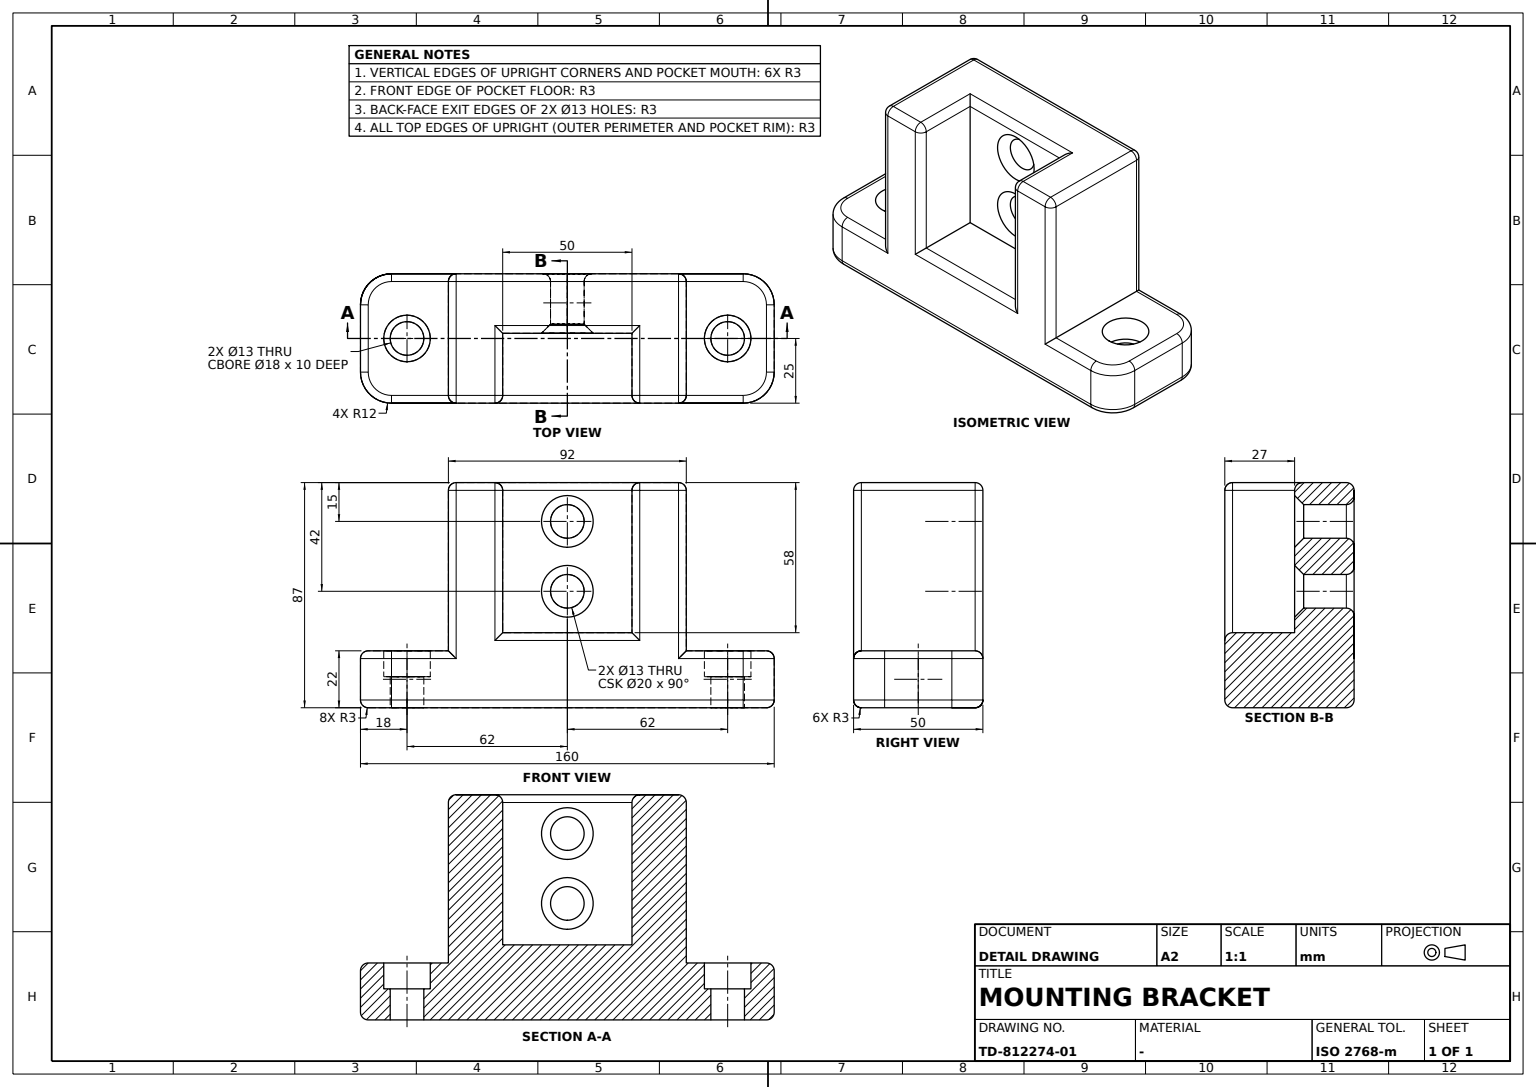
solid
v1 (-22,46,22)
v2 (-25,43,19)
e1 v1 v2 ELLIPSE(AX(P(-22,43,19),D(0,-0.707106781,0.707106781),D(0,-0.707106781,-0.707106781)),4.242641,3)
v3 (-25,43,84)
e2 v2 v3 LINE
v4 (-22,46,84)
e3 v3 v4 CIRCLE(AX(P(-22,43,84),D(0,0,1),D(1,0,0)),3) rev
e4 v1 v4 LINE
face CYL(AX(P(-22,43,42),D(0,0,1),D(-1,0,0)),3) [e1 e2 e3 -e4]
v5 (22,46,22)
v6 (25,43,19)
e5 v5 v6 ELLIPSE(AX(P(22,43,19),D(0,-0.707106781,0.707106781),D(0,0.707106781,0.707106781)),4.242641,3) rev
v7 (25,68,19)
e6 v7 v6 LINE
v8 (22,68,22)
e7 v7 v8 CIRCLE(AX(P(22,68,19),D(0,-1,0),D(0,0,-1)),3)
e8 v8 v5 LINE
face CYL(AX(P(22,0,19),D(0,-1,0),D(1,0,0)),3) [e5 -e6 e7 e8]
v9 (25,43,84)
v10 (22,46,84)
e9 v9 v10 CIRCLE(AX(P(22,43,84),D(0,0,1),D(1,0,0)),3)
e10 v6 v9 LINE
e11 v5 v10 LINE
face CYL(AX(P(22,43,42),D(0,0,1),D(1,0,0)),3) [-e9 -e10 -e5 e11]
v11 (25,-68,19)
v12 (22,-68,22)
e12 v11 v12 CIRCLE(AX(P(22,-68,19),D(0,-1,0),D(0,0,-1)),3)
v13 (25,-43,19)
e13 v13 v11 LINE
v14 (22,-46,22)
e14 v14 v13 ELLIPSE(AX(P(22,-43,19),D(0,-0.707106781,-0.707106781),D(0,-0.707106781,0.707106781)),4.242641,3) rev
e15 v14 v12 LINE
face CYL(AX(P(22,0,19),D(0,-1,0),D(1,0,0)),3) [-e12 -e13 -e14 e15]
v15 (22,-68,0)
v16 (25,-68,3)
e16 v15 v16 CIRCLE(AX(P(22,-68,3),D(0,1,0),D(0,0,1)),3) rev
v17 (22,68,0)
e17 v15 v17 LINE
v18 (25,68,3)
e18 v17 v18 CIRCLE(AX(P(22,68,3),D(0,1,0),D(0,0,1)),3) rev
e19 v16 v18 LINE
face CYL(AX(P(22,-8.4,3),D(0,1,0),D(0,0,-1)),3) [-e16 e17 e18 -e19]
v19 (22,25,84)
v20 (25,28,84)
e20 v19 v20 CIRCLE(AX(P(22,28,84),D(0,0,-1),D(-1,0,0)),3) rev
v21 (22,28,87)
e21 v20 v21 CIRCLE(AX(P(22,28,84),D(0,-1,0),D(0,0,-1)),3)
e22 v19 v21 CIRCLE(AX(P(22,28,84),D(-1,0,0),D(0,0,1)),3)
face SPHERE(AX(P(22,28,84),D(0,-1,0),D(0.997452115,0,-0.071339183)),3) [e20 e21 -e22]
v22 (-22,-46,84)
v23 (-22,-43,87)
e23 v22 v23 CIRCLE(AX(P(-22,-43,84),D(1,0,0),D(0,0,-1)),3) rev
v24 (22,-46,84)
e24 v22 v24 LINE
v25 (22,-43,87)
e25 v24 v25 CIRCLE(AX(P(22,-43,84),D(1,0,0),D(0,0,-1)),3) rev
e26 v23 v25 LINE
face CYL(AX(P(0,-43,84),D(1,0,0),D(0,-1,0)),3) [-e23 e24 e25 -e26]
v26 (-22,-46,22)
e27 v22 v26 LINE
e28 v26 v14 LINE
e29 v24 v14 LINE
face PLANE(AX(P(0,-46,22),D(0,1,0),D(0,0,1))) rev [-e24 e27 e28 -e29]
v27 (-13,77,0)
v28 (-13,80,3)
e30 v27 v28 CIRCLE(AX(P(-13,77,3),D(1,0,0),D(0,0,-1)),3)
v29 (-22,68,0)
e31 v29 v27 CIRCLE(AX(P(-13,68,0),D(0,0,-1),D(-1,0,0)),9)
v30 (-25,68,3)
e32 v29 v30 CIRCLE(AX(P(-22,68,3),D(0,-1,0),D(0,0,-1)),3) rev
e33 v30 v28 CIRCLE(AX(P(-13,68,3),D(0,0,1),D(1,0,0)),12) rev
face TORUS(AX(P(-13,68,3),D(0,0,-1),D(-0.163937522,-0.986470724,0)),9,3) [-e30 -e31 e32 e33]
v31 (9,-62,22)
e34 v31 v31 CIRCLE(AX(P(0,-62,22),D(0,0,1),D(1,0,0)),9)
v32 (13,-77,22)
e35 v32 v12 CIRCLE(AX(P(13,-68,22),D(0,0,1),D(1,0,0)),9)
v33 (-22,-68,22)
e36 v26 v33 LINE
v34 (-13,-77,22)
e37 v33 v34 CIRCLE(AX(P(-13,-68,22),D(0,0,1),D(1,0,0)),9)
e38 v34 v32 LINE
face PLANE(AX(P(0,80,22),D(0,0,1),D(0,-1,0))) [-e34] [e35 -e15 -e28 e36 e37 e38]
v35 (-2,-25,84)
v36 (-5,-28,87)
e39 v35 v36 ELLIPSE(AX(P(-5,-28,84),D(-0.707106781,0.707106781,0),D(0.707106781,0.707106781,0)),4.242641,3) rev
v37 (-2,25,84)
e40 v35 v37 LINE
v38 (-5,28,87)
e41 v37 v38 ELLIPSE(AX(P(-5,28,84),D(-0.707106781,-0.707106781,0),D(-0.707106781,0.707106781,0)),4.242641,3)
e42 v36 v38 LINE
face CYL(AX(P(-5,0,84),D(0,1,0),D(1,0,0)),3) [-e39 e40 e41 -e42]
v39 (25,-43,84)
e43 v39 v25 CIRCLE(AX(P(22,-43,84),D(0,-1,0),D(0,0,-1)),3)
e44 v24 v39 CIRCLE(AX(P(22,-43,84),D(0,0,-1),D(-1,0,0)),3) rev
face SPHERE(AX(P(22,-43,84),D(0,-1,0),D(0.997452115,0,-0.071339183)),3) [e43 -e25 e44]
v40 (22,43,87)
e45 v40 v10 CIRCLE(AX(P(22,43,84),D(1,0,0),D(0,0,-1)),3) rev
e46 v9 v40 CIRCLE(AX(P(22,43,84),D(0,-1,0),D(0,0,-1)),3)
face SPHERE(AX(P(22,43,84),D(0,1,0),D(0.997452115,0,-0.071339183)),3) [-e45 -e46 e9]
v41 (25,-28,84)
v42 (22,-28,87)
e47 v41 v42 CIRCLE(AX(P(22,-28,84),D(0,-1,0),D(0,0,-1)),3)
e48 v42 v25 LINE
e49 v41 v39 LINE
face CYL(AX(P(22,0,84),D(0,-1,0),D(0,0,1)),3) [e47 e48 -e43 -e49]
v43 (25,-28,26)
e50 v43 v41 LINE
v44 (22,-25,29)
e51 v44 v43 ELLIPSE(AX(P(22,-28,26),D(0,-0.707106781,0.707106781),D(0,0.707106781,0.707106781)),4.242641,3) rev
v45 (22,-25,84)
e52 v44 v45 LINE
e53 v45 v41 CIRCLE(AX(P(22,-28,84),D(0,0,1),D(1,0,0)),3) rev
face CYL(AX(P(22,-28,42),D(0,0,1),D(0,1,0)),3) [-e50 -e51 e52 e53]
v46 (13,-80,19)
e54 v46 v32 CIRCLE(AX(P(13,-77,19),D(1,0,0),D(0,0,-1)),3) rev
e55 v46 v11 CIRCLE(AX(P(13,-68,19),D(0,0,1),D(1,0,0)),12)
face TORUS(AX(P(13,-68,19),D(0,0,1),D(-0.988441034,-0.151605813,0)),9,3) [e12 -e35 -e54 e55]
v47 (-22,-68,0)
e56 v29 v47 LINE
v48 (-25,-68,3)
e57 v47 v48 CIRCLE(AX(P(-22,-68,3),D(0,-1,0),D(0,0,-1)),3) rev
e58 v30 v48 LINE
face CYL(AX(P(-22,8.4,3),D(0,-1,0),D(0,0,-1)),3) [-e32 e56 e57 -e58]
v49 (-9,62,12)
e59 v49 v49 CIRCLE(AX(P(0,62,12),D(0,0,-1),D(-1,0,0)),9)
v50 (-6.5,62,12)
e60 v50 v50 CIRCLE(AX(P(0,62,12),D(0,0,-1),D(-1,0,0)),6.5)
face PLANE(AX(P(6.5,62,12),D(0,0,-1),D(1,0,0))) rev [-e59] [e60]
v51 (-22,0,78.5)
e61 v51 v51 CIRCLE(AX(P(-22,0,72),D(-1,0,0),D(0,0,1)),6.5) rev
v52 (-25,0,62.5)
e62 v52 v52 CIRCLE(AX(P(-25,0,72),D(1,0,0),D(0,0,-1)),9.5)
face TORUS(AX(P(-22,0,72),D(1,0,0),D(0,0.208573787,-0.978006634)),9.5,3) [e61] [-e62]
v53 (13,80,3)
v54 (13,80,19)
e63 v53 v54 LINE
e64 v7 v54 CIRCLE(AX(P(13,68,19),D(0,0,1),D(1,0,0)),12)
e65 v18 v7 LINE
e66 v53 v18 CIRCLE(AX(P(13,68,3),D(0,0,1),D(1,0,0)),12) rev
face CYL(AX(P(13,68,43.5),D(0,0,1),D(0,1,0)),12) [e63 -e64 -e65 -e66]
v55 (-25,-68,19)
e67 v48 v55 LINE
v56 (-13,-80,3)
e68 v56 v48 CIRCLE(AX(P(-13,-68,3),D(0,0,1),D(1,0,0)),12) rev
v57 (-13,-80,19)
e69 v56 v57 LINE
e70 v55 v57 CIRCLE(AX(P(-13,-68,19),D(0,0,1),D(1,0,0)),12)
face CYL(AX(P(-13,-68,43.5),D(0,0,1),D(-1,0,0)),12) [-e67 -e68 e69 -e70]
v58 (9,62,22)
e71 v58 v58 CIRCLE(AX(P(0,62,22),D(0,0,1),D(1,0,0)),9)
face CYL(AX(P(0,62,21.9),D(0,0,-1),D(1,0,0)),9) rev [e59] [e71]
e72 v4 v10 LINE
e73 v1 v5 LINE
face PLANE(AX(P(0,46,22),D(0,1,0),D(0,0,1))) [e72 -e11 -e73 e4]
v59 (13,-80,3)
e74 v59 v46 LINE
e75 v16 v59 CIRCLE(AX(P(13,-68,3),D(0,0,1),D(1,0,0)),12) rev
e76 v16 v11 LINE
face CYL(AX(P(13,-68,43.5),D(0,0,1),D(0,-1,0)),12) [-e74 -e75 e76 -e55]
v60 (-22,43,87)
e77 v60 v3 CIRCLE(AX(P(-22,43,84),D(0,-1,0),D(0,0,-1)),3)
e78 v60 v4 CIRCLE(AX(P(-22,43,84),D(1,0,0),D(0,0,-1)),3) rev
face SPHERE(AX(P(-22,43,84),D(0,1,0),D(0.071339183,0,0.997452115)),3) [-e77 e78 -e3]
v61 (-6.5,-62,12)
e79 v61 v61 CIRCLE(AX(P(0,-62,12),D(0,0,-1),D(-1,0,0)),6.5)
v62 (-6.5,-62,0)
e80 v62 v62 CIRCLE(AX(P(0,-62,0),D(0,0,-1),D(-1,0,0)),6.5)
face CYL(AX(P(0,-62,21.9),D(0,0,-1),D(1,0,0)),6.5) rev [-e79] [e80]
e81 v28 v53 LINE
v63 (-13,80,19)
e82 v28 v63 LINE
e83 v63 v54 LINE
face PLANE(AX(P(0,80,0),D(0,1,0),D(0,0,1))) [-e63 -e81 e82 e83]
e84 v60 v23 LINE
v64 (-25,-43,84)
e85 v3 v64 LINE
e86 v23 v64 CIRCLE(AX(P(-22,-43,84),D(0,-1,0),D(0,0,-1)),3)
face CYL(AX(P(-22,0,84),D(0,-1,0),D(-1,0,0)),3) [-e84 e77 e85 -e86]
e87 v9 v20 LINE
v65 (25,28,26)
e88 v20 v65 LINE
e89 v65 v43 LINE
e90 v39 v13 LINE
face PLANE(AX(P(25,0,0),D(1,0,0),D(0,1,0))) [e87 e88 e89 e50 e49 e90 e13 -e76 e19 e65 e6 e10]
e91 v40 v21 LINE
face CYL(AX(P(22,0,84),D(0,-1,0),D(0,0,1)),3) [e46 e91 -e21 -e87]
v66 (-2,-25,29)
e92 v66 v35 LINE
v67 (-2,25,29)
e93 v67 v66 LINE
e94 v37 v67 LINE
v68 (-2,0,62)
e95 v68 v68 CIRCLE(AX(P(-2,0,72),D(1,0,0),D(0,0,-1)),10)
v69 (-2,0,35)
e96 v69 v69 CIRCLE(AX(P(-2,0,45),D(1,0,0),D(0,0,-1)),10)
face PLANE(AX(P(-2,0,0),D(1,0,0),D(0,1,0))) [-e92 -e93 -e94 -e40] [-e95] [-e96]
v70 (13,-77,0)
e97 v15 v70 CIRCLE(AX(P(13,-68,0),D(0,0,-1),D(-1,0,0)),9)
e98 v70 v59 CIRCLE(AX(P(13,-77,3),D(1,0,0),D(0,0,-1)),3) rev
face TORUS(AX(P(13,-68,3),D(0,0,-1),D(0.163937522,0.986470724,0)),9,3) [-e97 e16 e75 -e98]
e99 v45 v35 LINE
e100 v42 v36 LINE
e101 v45 v42 CIRCLE(AX(P(22,-28,84),D(-1,0,0),D(0,0,1)),3) rev
face CYL(AX(P(0,-28,84),D(-1,0,0),D(0,1,0)),3) [e99 e39 -e100 -e101]
e102 v21 v38 LINE
e103 v60 v40 LINE
face PLANE(AX(P(0,46,87),D(0,0,1),D(0,-1,0))) [e100 e42 -e102 -e91 -e103 e84 e26 -e48]
face CYL(AX(P(22,-43,42),D(0,0,-1),D(0,-1,0)),3) [e14 -e90 -e44 e29]
v71 (-22,0,51.5)
e104 v71 v71 CIRCLE(AX(P(-22,0,45),D(-1,0,0),D(0,0,1)),6.5) rev
v72 (-25,0,35.5)
e105 v72 v72 CIRCLE(AX(P(-25,0,45),D(1,0,0),D(0,0,-1)),9.5)
face TORUS(AX(P(-22,0,45),D(1,0,0),D(0,0.208573787,-0.978006634)),9.5,3) [e104] [-e105]
v73 (13,77,22)
e106 v54 v73 CIRCLE(AX(P(13,77,19),D(1,0,0),D(0,0,-1)),3)
e107 v8 v73 CIRCLE(AX(P(13,68,22),D(0,0,1),D(1,0,0)),9)
face TORUS(AX(P(13,68,19),D(0,0,1),D(0.151605813,-0.988441034,0)),9,3) [e64 e106 -e107 -e7]
v74 (22,25,29)
e108 v74 v65 ELLIPSE(AX(P(22,28,26),D(0,-0.707106781,-0.707106781),D(0,-0.707106781,0.707106781)),4.242641,3) rev
e109 v19 v74 LINE
face CYL(AX(P(22,28,42),D(0,0,-1),D(0,-1,0)),3) [e108 -e88 -e20 e109]
v75 (-5.5,0,38.5)
e110 v75 v75 CIRCLE(AX(P(-5.5,0,45),D(1,0,0),D(0,0,-1)),6.5) rev
face CYL(AX(P(-2.1,0,45),D(-1,0,0),D(0,1,0)),6.5) rev [-e104] [-e110]
face SPHERE(AX(P(22,-28,84),D(0,1,0),D(0.997452115,0,-0.071339183)),3) [-e53 e101 -e47]
v76 (-25,-43,19)
e111 v26 v76 ELLIPSE(AX(P(-22,-43,19),D(0,-0.707106781,-0.707106781),D(0,0.707106781,-0.707106781)),4.242641,3)
e112 v76 v55 LINE
e113 v55 v33 CIRCLE(AX(P(-22,-68,19),D(0,-1,0),D(0,0,-1)),3) rev
face CYL(AX(P(-22,0,19),D(0,-1,0),D(-1,0,0)),3) [-e36 e111 e112 e113]
v77 (-25,68,19)
e114 v77 v2 LINE
v78 (-22,68,22)
e115 v78 v1 LINE
e116 v77 v78 CIRCLE(AX(P(-22,68,19),D(0,-1,0),D(0,0,-1)),3) rev
face CYL(AX(P(-22,0,19),D(0,-1,0),D(-1,0,0)),3) [e114 -e1 -e115 -e116]
v79 (-13,77,22)
e117 v79 v73 LINE
e118 v79 v78 CIRCLE(AX(P(-13,68,22),D(0,0,1),D(1,0,0)),9)
face PLANE(AX(P(0,80,22),D(0,0,1),D(0,-1,0))) [-e71] [e107 -e117 e118 e115 e73 -e8]
v80 (-5.5,0,65.5)
e119 v80 v80 CIRCLE(AX(P(-5.5,0,72),D(1,0,0),D(0,0,-1)),6.5) rev
face CONE(AX(P(-5.5,0,72),D(1,0,0),D(0,1,0)),6.5,0.785398163) rev [e119] [e95]
e120 v30 v77 LINE
e121 v63 v77 CIRCLE(AX(P(-13,68,19),D(0,0,1),D(1,0,0)),12)
face CYL(AX(P(-13,68,43.5),D(0,0,1),D(-1,0,0)),12) [e120 -e121 -e82 -e33]
v81 (13,77,0)
e122 v81 v17 CIRCLE(AX(P(13,68,0),D(0,0,-1),D(-1,0,0)),9)
e123 v81 v53 CIRCLE(AX(P(13,77,3),D(1,0,0),D(0,0,-1)),3)
face TORUS(AX(P(13,68,3),D(0,0,-1),D(-0.986470724,0.163937522,0)),9,3) [-e18 -e122 e123 e66]
e124 v63 v79 CIRCLE(AX(P(-13,77,19),D(1,0,0),D(0,0,-1)),3)
face CYL(AX(P(0,77,19),D(1,0,0),D(0,1,0)),3) [-e83 e124 e117 -e106]
e125 v57 v34 CIRCLE(AX(P(-13,-77,19),D(1,0,0),D(0,0,-1)),3) rev
face TORUS(AX(P(-13,-68,19),D(0,0,1),D(-0.151605813,0.988441034,0)),9,3) [-e37 -e113 e70 e125]
v82 (-6.5,62,0)
e126 v82 v82 CIRCLE(AX(P(0,62,0),D(0,0,-1),D(-1,0,0)),6.5)
face CYL(AX(P(0,62,21.9),D(0,0,-1),D(1,0,0)),6.5) rev [-e60] [e126]
e127 v22 v64 CIRCLE(AX(P(-22,-43,84),D(0,0,-1),D(-1,0,0)),3)
face SPHERE(AX(P(-22,-43,84),D(0,-1,0),D(0.071339183,0,0.997452115)),3) [e86 -e127 e23]
face CONE(AX(P(-5.5,0,45),D(1,0,0),D(0,1,0)),6.5,0.785398163) rev [e110] [e96]
e128 v27 v81 LINE
face CYL(AX(P(0,77,3),D(1,0,0),D(0,0,-1)),3) [-e123 -e128 e30 e81]
v83 (-9,-62,12)
e129 v83 v83 CIRCLE(AX(P(0,-62,12),D(0,0,-1),D(-1,0,0)),9)
face PLANE(AX(P(6.5,62,12),D(0,0,-1),D(1,0,0))) rev [-e129] [e79]
e130 v64 v76 LINE
face PLANE(AX(P(-25,0,0),D(1,0,0),D(0,1,0))) rev [-e114 -e120 e58 e67 -e112 -e130 -e85 -e2] [e62] [e105]
face CYL(AX(P(-22,-43,42),D(0,0,-1),D(0,-1,0)),3) [e130 -e111 -e27 e127]
e131 v56 v59 LINE
e132 v57 v46 LINE
face PLANE(AX(P(0,-80,0),D(0,1,0),D(0,0,1))) rev [-e69 e131 e74 -e132]
v84 (-13,-77,0)
e133 v84 v56 CIRCLE(AX(P(-13,-77,3),D(1,0,0),D(0,0,-1)),3) rev
e134 v84 v70 LINE
face CYL(AX(P(0,-77,3),D(1,0,0),D(0,0,-1)),3) [-e131 -e133 e134 e98]
e135 v44 v66 LINE
face PLANE(AX(P(25,-25,29),D(0,-1,0),D(0,0,1))) rev [e92 -e99 -e52 e135]
face CYL(AX(P(0,-77,19),D(1,0,0),D(0,-1,0)),3) [-e38 -e125 e132 e54]
face CYL(AX(P(0,43,84),D(1,0,0),D(0,0,1)),3) [-e78 e103 e45 -e72]
e136 v74 v67 LINE
e137 v19 v37 LINE
face PLANE(AX(P(25,25,87),D(0,1,0),D(0,0,-1))) rev [e94 -e136 -e109 e137]
face CYL(AX(P(-2.1,0,72),D(-1,0,0),D(0,1,0)),6.5) rev [-e119] [-e61]
e138 v74 v44 LINE
face CYL(AX(P(22,0,26),D(0,-1,0),D(1,0,0)),3) [e51 -e89 -e108 e138]
e139 v84 v47 CIRCLE(AX(P(-13,-68,0),D(0,0,-1),D(-1,0,0)),9)
face TORUS(AX(P(-13,-68,3),D(0,0,-1),D(0.986470724,-0.163937522,0)),9,3) [-e139 e133 e68 -e57]
face CYL(AX(P(0,28,84),D(-1,0,0),D(0,-1,0)),3) [-e137 e22 e102 -e41]
face CYL(AX(P(0,-62,21.9),D(0,0,-1),D(1,0,0)),9) rev [e34] [e129]
face PLANE(AX(P(25,25,29),D(0,0,-1),D(0,-1,0))) rev [-e135 -e138 e136 e93]
face PLANE(AX(P(0,-80,0),D(0,0,-1),D(0,1,0))) [-e80] [-e126] [e97 -e134 e139 -e56 e31 e128 e122 -e17]
face TORUS(AX(P(-13,68,19),D(0,0,1),D(0.988441034,0.151605813,0)),9,3) [-e124 e121 e116 -e118]
